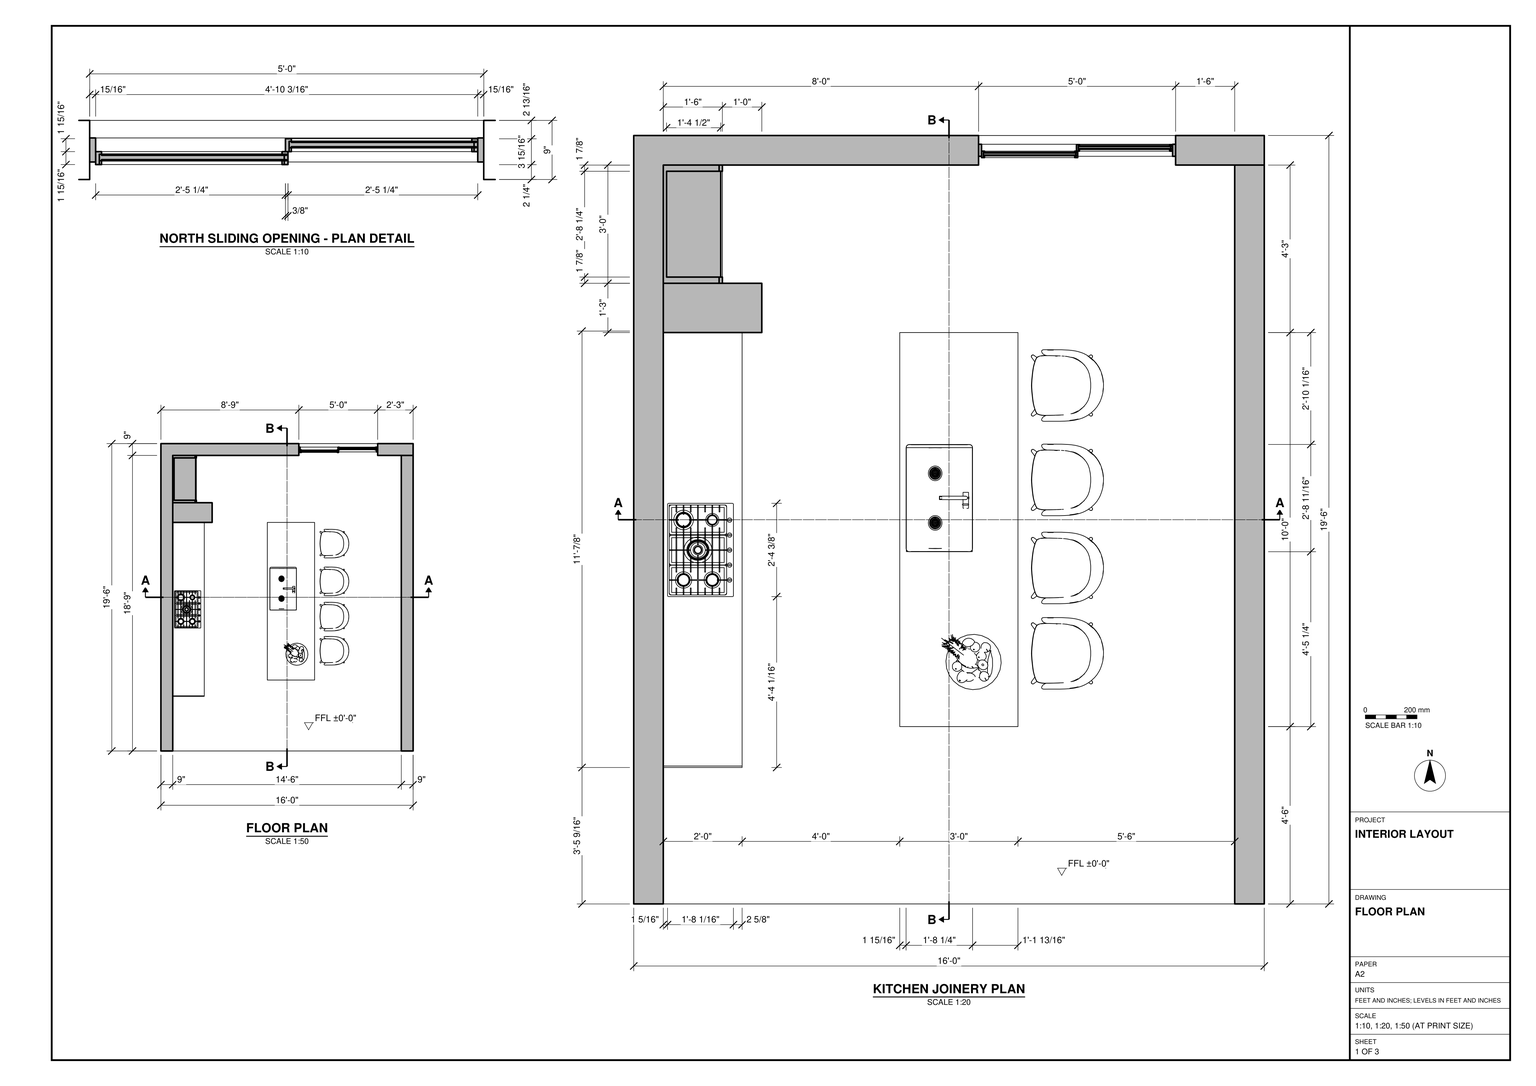
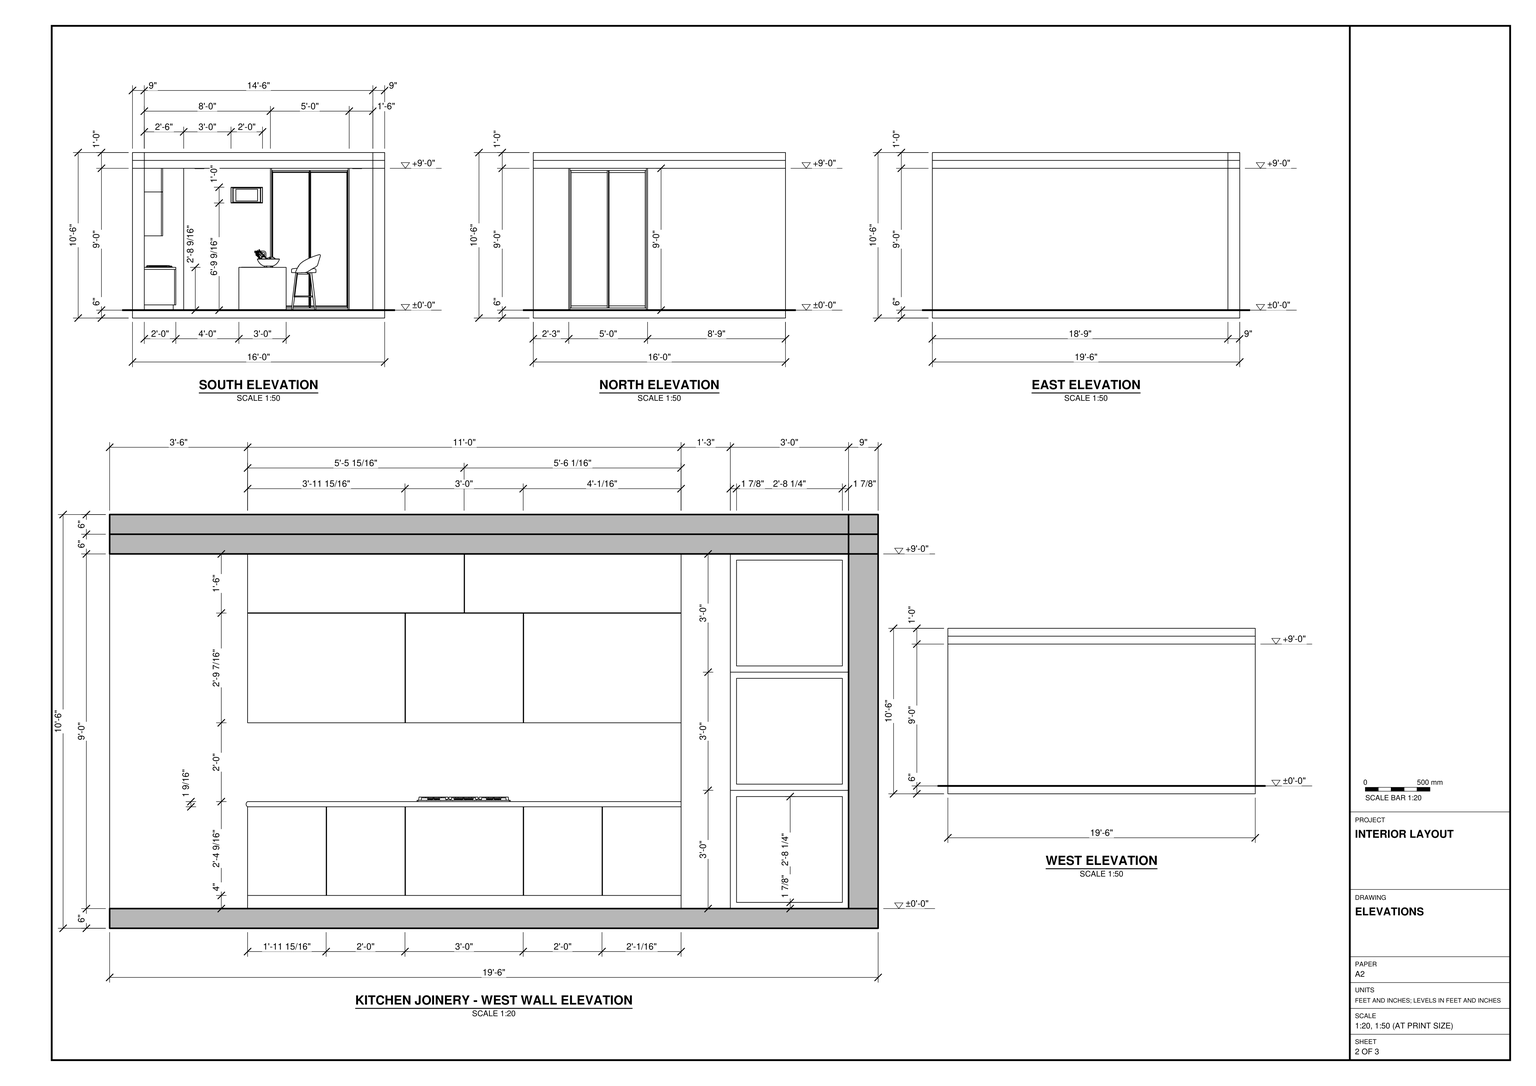
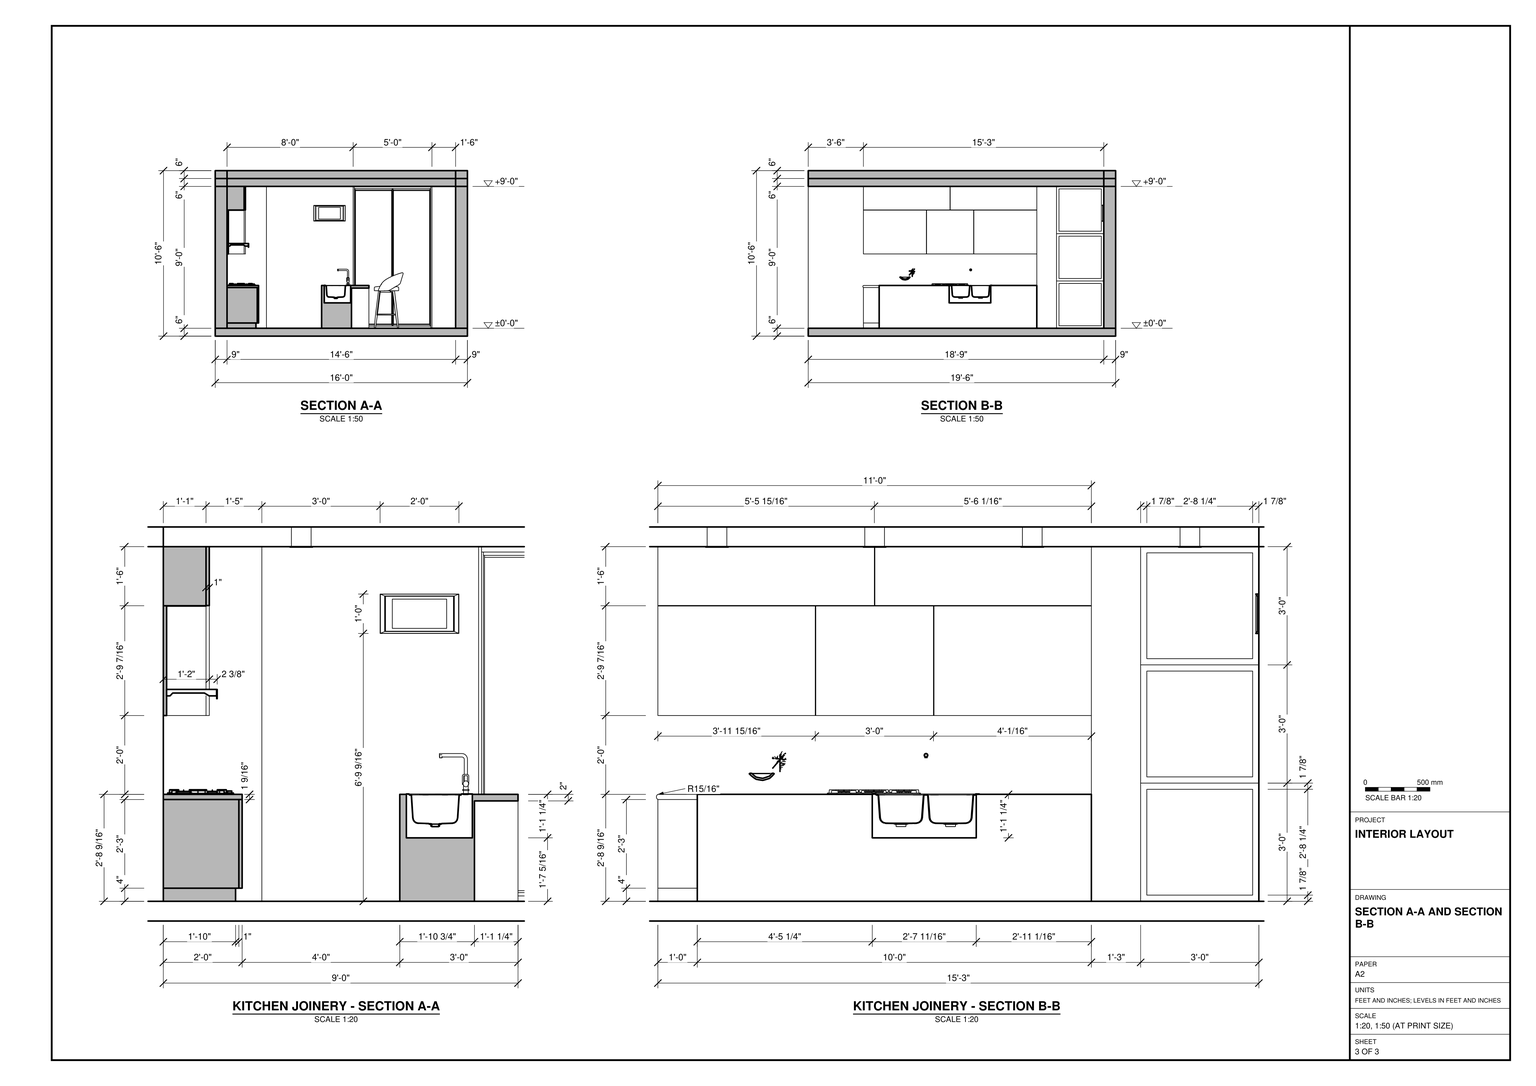
Use task_files/diagram_01.pdf to model the kitchen in SketchUp. Work in feet and inches. Set the finished floor at ±0'-0". The shell measures 16'-0" east to west by 19'-6" north to south and is 10'-6" high overall. Model the floor slab, the 9" walls on the west, north and east sides, and the flat ceiling and roof assembly shown in section. Leave the south side open. Use the enlarged plan detail for the two sliding panels in the north wall.

Build the west counter run with its recessed toe kick, divided cabinet fronts, cooktop and wall cabinets. Follow the west wall elevation for the two rows of upper cabinet fronts and the separate full-height storage at the north end. Set the island parallel to the counter, leaving a 4'-0" working aisle. Use the sections to position the double-bowl sink and tap and to form the overhang for the four stools on the east side. Place the fruit bowl near the south end of the island.

Keep the shell elements and each furniture or joinery piece in separate groups or components, and use components for repeated parts. Decor and loose items, including appliances, may be any suitable library components. Save one SketchUp model as output_files/kitchen_with_wall_cabinets_and_a_sink_island.skp.

# SketchUp Ruby script. Lengths in inches.
U = 1.inch
M = Sketchup.active_model
def pt(a) = Geom::Point3d.new(a.map { |v| v * U })
def face(e, loops, mat)
  f = e.add_face(loops[0].map { |a| pt(a) })
  loops[1..].each { |l| e.add_face(l.map { |a| pt(a) }).erase! }
  f.material = f.back_material = mat if mat
  f
end
# faces: each face lists its corners as indices into pts; further lists are holes
def faces(e, pts, list, mat = nil) = list.each { |f| face(e, (f[0].is_a?(Array) ? f : [f]).map { |l| l.map { |i| pts[i] } }, mat) }
# xy, xz, yz: faces in a plane at the given z, y or x. An outline is a flat list of corners, or four numbers for a rectangle; further outlines are holes
def ring(l) = l.size == 4 ? [[l[0], l[1]], [l[2], l[1]], [l[2], l[3]], [l[0], l[3]]] : l.each_slice(2).to_a
def flat(e, list, mat, &to3) = list.each { |f| face(e, (f[0].is_a?(Array) ? f : [f]).map { |l| ring(l).map { |u, v| to3.(u, v) } }, mat) }
def xy(e, z, list, mat = nil) = flat(e, list, mat) { |x, y| [x, y, z] }
def xz(e, y, list, mat = nil) = flat(e, list, mat) { |x, z| [x, y, z] }
def yz(e, x, list, mat = nil) = flat(e, list, mat) { |y, z| [x, y, z] }
def lines(e, pts, list) = list.each { |a, b| e.add_line(pt(pts[a]), pt(pts[b])) }
# prism: a flat outline (further loops are holes) pulled along v
def prism(e, loops, v, mat = nil)
  f = face(e, loops, mat); d = Geom::Vector3d.new(v.map { |x| x * U })
  f.pushpull(f.normal.samedirection?(d) ? d.length : -d.length)
end
def box(e, o, s, mat = nil) = prism(e, [[o, [o[0] + s[0], o[1], o[2]], [o[0] + s[0], o[1] + s[1], o[2]], [o[0], o[1] + s[1], o[2]]]], [0, 0, s[2]], mat)
def at(x, y, z, deg = 0) = Geom::Transformation.translation(pt([x, y, z])) * Geom::Transformation.rotation(ORIGIN, Z_AXIS, deg.degrees)
def axes(o, x, y, z) = Geom::Transformation.new([*x, 0, *y, 0, *z, 0, *pt(o).to_a, 1])
def part(name) = M.definitions.add(name)
# library, detail: a bought-in or finely detailed component or shape, given as its bounding box
def library(name, o, s) = part(name).tap { |d| box(d.entities, o, s) }
def detail(e, o, s) = box(e.add_group.entities, o, s)
def put(e, d, t, mat = nil) = e.add_instance(d, t).tap { |i| i.material = mat if mat }
def group(e, t, mat = nil) = e.add_group.tap { |g| g.transformation = t; g.material = mat if mat }.entities
root = M.entities
M.materials.add("Calacatta Marble (Y7X0XK)").color = [232, 232, 228]
M.materials.add("Charred Timber (ZWV9ZF)").color = [34, 34, 33]
M.materials.add("Resene FilmPro White -").color = [250, 246, 236]
M.materials.add("[0128_White]").color = [255, 255, 255]
M.materials.add("[0135_DarkGray]").color = [81, 81, 81]
M.materials.add("[Translucent Glass Gray]").color = [128, 128, 128]
M.materials["[Translucent Glass Gray]"].alpha = 0.5
M.materials.add("[Translucent Glass Gray]1").color = [128, 128, 128]
M.materials["[Translucent Glass Gray]1"].alpha = 0.15
c1 = library("Chimney",[0,-0.01,0],[29.73,15.52,29.75])
c2 = library("Piano cottura 702",[-24.9,5.55,2.1875],[20.06,28.4,1.39])
c3 = library("MIRELLA BAR HARD 7 colors",[-10.9,-9.34,0],[21.81,22.01,42.29])
c4 = library("Template",[-17.21,0.04,0.05],[27.44,26.51,14.69])
c5 = part("OA3")
g1 = group(c5.entities,at(77.64,-15.68,17.68))
prism(g1,[[[0.35,42.52,3.15],[0.35,42.52,51.84],[0.35,3.15,51.84],[0.35,3.15,3.15]],[[0.35,38.58,7.09],[0.35,7.09,7.09],[0.35,7.09,47.91],[0.35,38.58,47.91]]],[-0.35,0,0],"[0128_White]")
g2 = group(g1,at(1.57,0,0,90))
xy(g2,0,[[0,0,26.23,1.57],[26.23,0,45.67,1.57]],"Resene FilmPro White -")
xy(g2,0.2,[[0.2,0,45.47,0.12]],"Resene FilmPro White -")
xy(g2,2.64,[[2.64,0.71,43.03,0.83]],"Resene FilmPro White -")
xy(g2,2.76,[[2.76,0.83,42.91,0.94]],"Resene FilmPro White -")
xy(g2,3.03,[[3.03,0.94,42.64,1.0625]],"Resene FilmPro White -")
xy(g2,3.15,[[3.15,1.0625,42.52,1.57]],"Resene FilmPro White -")
xy(g2,51.84,[[3.15,1.0625,42.52,1.57]],"Resene FilmPro White -")
xy(g2,51.96,[[3.03,0.94,42.64,1.0625]],"Resene FilmPro White -")
xy(g2,52.24,[[2.76,0.83,42.91,0.94]],"Resene FilmPro White -")
xy(g2,52.35,[[2.64,0.71,43.03,0.83]],"Resene FilmPro White -")
xy(g2,54.8,[[0.2,0,45.47,0.12]],"Resene FilmPro White -")
xy(g2,54.99,[[0,0,45.67,1.57]],"Resene FilmPro White -")
xz(g2,0,[[[0,0,45.67,54.99],[0.2,0.2,45.47,54.8]]],"Resene FilmPro White -")
xz(g2,0.83,[[[2.64,2.64,43.03,52.35],[2.76,2.76,42.91,52.24]]],"Resene FilmPro White -")
xz(g2,0.94,[[[2.76,2.76,42.91,52.24],[3.03,3.03,42.64,51.96]]],"Resene FilmPro White -")
xz(g2,1.0625,[[[3.03,3.03,42.64,51.96],[3.15,3.15,42.52,51.84]]],"Resene FilmPro White -")
xz(g2,1.57,[[[0,0,45.67,54.99],[3.15,3.15,42.52,51.84]]],"Resene FilmPro White -")
yz(g2,0,[[0,0,1.57,54.99]],"Resene FilmPro White -")
yz(g2,0.2,[[0,0.2,0.12,54.8]],"Resene FilmPro White -")
yz(g2,2.64,[[0.71,2.64,0.83,52.35]],"Resene FilmPro White -")
yz(g2,2.76,[[0.83,2.76,0.94,52.24]],"Resene FilmPro White -")
yz(g2,3.03,[[0.94,3.03,1.0625,51.96]],"Resene FilmPro White -")
yz(g2,3.15,[[1.0625,3.15,1.57,51.84]],"Resene FilmPro White -")
yz(g2,42.52,[[1.0625,3.15,1.57,51.84]],"Resene FilmPro White -")
yz(g2,42.64,[[0.94,3.03,1.0625,51.96]],"Resene FilmPro White -")
yz(g2,42.91,[[0.83,2.76,0.94,52.24]],"Resene FilmPro White -")
yz(g2,43.03,[[0.71,2.64,0.83,52.35]],"Resene FilmPro White -")
yz(g2,45.47,[[0,0.2,0.12,54.8]],"Resene FilmPro White -")
yz(g2,45.67,[[0,0,1.57,54.99]],"Resene FilmPro White -")
p = [[2.64,0.71,52.35],[0.2,0.12,54.8],[0.2,0.12,0.2],[2.64,0.71,2.64],[45.47,0.12,0.2],[43.03,0.71,2.64],
  [45.47,0.12,54.8],[43.03,0.71,52.35]]
faces(g2,p,[[0,1,2,3],[3,2,4,5],[5,4,6,7],[7,6,1,0]],"Resene FilmPro White -")
c6 = library("sink",[0,0,0],[20.24,32.66,22.26])
c7 = part("PENTEK_RP Fineline 50S_Sliding_DoorCase_E1")
box(c7.entities,[0,0,0],[1.51,3.66,99.27],"[0135_DarkGray]")
c8 = part("PENTEK_RP Fineline 50S_SlidingDooe_Case_E2")
box(c8.entities,[0,0,0],[96.25,3.66,1.51],"[0135_DarkGray]")
c9 = part("pentek_RP Fineline 50S_SlidingDoor_Case")
put(c9.entities,c7,at(97.76,0,0))
put(c9.entities,c8,at(1.51,0,0))
put(c9.entities,c7,at(0,0,0))
put(c9.entities,c8,at(1.51,0,97.76))
c10 = part("PENTEK_RP Fineline 50S_SlidingDoor_GlazingBead_2")
box(c10.entities,[0,0,0],[0.56,0.59,94.39],"[0135_DarkGray]")
c11 = part("PENTEK_RP Fineline 50S_SlidingDoor_Glass")
box(c11.entities,[0,0,0],[46.58,0.16,94.39],"[Translucent Glass Gray]1")
c12 = part("PENTEK_RP Fineline 50S_SlidingDoor_GlazingBead")
box(c12.entities,[0,0,0],[45.47,0.59,0.56],"[0135_DarkGray]")
c13 = part("PENTEK_RP Fineline 50S_SlidingDoor_Leaf_E1")
xy(c13.entities,0,[[0,0,0.93,1.97],[0.93,1.57,1.49,1.97]],"[0135_DarkGray]")
xy(c13.entities,96.25,[[0,0,0.93,0,0.93,1.57,1.49,1.57,1.49,1.97,0,1.97]],"[0135_DarkGray]")
xz(c13.entities,0,[[0,0,0.93,96.25]],"[0135_DarkGray]")
xz(c13.entities,1.57,[[0.93,0,1.49,95.32],[0.93,95.32,1.49,96.25]],"[0135_DarkGray]")
xz(c13.entities,1.97,[[0,0,1.49,96.25]],"[0135_DarkGray]")
yz(c13.entities,0,[[0,0,1.97,96.25]],"[0135_DarkGray]")
yz(c13.entities,0.93,[[0,0,1.57,0.93],[0,0.93,1.57,95.32],[0,95.32,1.57,96.25]],"[0135_DarkGray]")
yz(c13.entities,1.49,[[1.57,0,1.97,95.32],[1.57,95.32,1.97,96.25]],"[0135_DarkGray]")
c14 = part("PENTEK_RP Fineline 50S_SlidingDoor_Leaf_E2")
xy(c14.entities,0,[[0,0,0,1.57,0.56,1.57,0.56,1.97,46.02,1.97,46.02,1.57,46.58,1.57,46.58,0]],"[0135_DarkGray]")
xy(c14.entities,0.93,[[0,0,46.58,1.57]],"[0135_DarkGray]")
xy(c14.entities,1.49,[[0.56,1.57,46.02,1.97]],"[0135_DarkGray]")
xz(c14.entities,0,[[0,0,46.58,0.93]],"[0135_DarkGray]")
xz(c14.entities,1.57,[[0,0,0.56,0.93],[46.02,0,46.58,0.93],[0.56,0.93,46.02,1.49]],"[0135_DarkGray]")
xz(c14.entities,1.97,[[0.56,0,46.02,1.49]],"[0135_DarkGray]")
yz(c14.entities,0,[[0,0,1.57,0.93]],"[0135_DarkGray]")
yz(c14.entities,0.56,[[1.57,0,1.97,0.93],[1.57,0.93,1.97,1.49]],"[0135_DarkGray]")
yz(c14.entities,46.02,[[1.57,0,1.97,0.93],[1.57,0.93,1.97,1.49]],"[0135_DarkGray]")
yz(c14.entities,46.58,[[0,0,1.57,0.93]],"[0135_DarkGray]")
c15 = part("PENTEK_RP Fineline S_SlidingDoor_Leaf1")
put(c15.entities,c10,at(0.93,0,0.93))
put(c15.entities,c10,at(46.96,0,0.93))
put(c15.entities,c11,at(1.49,1.42,0.93))
put(c15.entities,c12,at(1.49,0,0.93))
put(c15.entities,c11,at(1.49,0.59,0.93))
put(c15.entities,c13,at(0,0,0))
put(c15.entities,c13,axes([48.44,0,0],[-1,0,0],[0,1,0],[0,0,1]))
put(c15.entities,c14,axes([0.93,0,96.25],[1,0,0],[0,1,0],[0,0,-1]))
put(c15.entities,c14,at(0.93,0,0))
put(c15.entities,c12,at(1.49,0,94.77))
c16 = part("PENTEK_RP Fineline 50S_SlidingDoor_Leaf2")
put(c16.entities,c11,at(1.49,1.42,0.93))
put(c16.entities,c12,at(1.49,0,94.77))
put(c16.entities,c10,at(46.96,0,0.93))
put(c16.entities,c11,at(1.49,0.59,0.93))
put(c16.entities,c10,at(0.93,0,0.93))
put(c16.entities,c13,at(0,0,0))
put(c16.entities,c13,axes([48.44,0,0],[-1,0,0],[0,1,0],[0,0,1]))
put(c16.entities,c12,at(1.49,0,0.93))
put(c16.entities,c14,axes([0.93,0,96.25],[1,0,0],[0,1,0],[0,0,-1]))
put(c16.entities,c14,at(0.93,0,0))
c17 = part("PENTEK_RP+Fineline+50S_Sliding_Door+(1)")
put(c17.entities,c9,at(0,-1.88,-0.09))
put(c17.entities,c15,at(1.51,-2.27,1.42))
put(c17.entities,c16,at(49.32,-0.3,1.42))
c18 = part("Side plate")
xy(c18.entities,-0.25,[[[2.99,-0.5,2.09,-0.38,1.24,-0.03,0.52,0.53,-0.03,1.26,-0.38,2.1,-0.5,3.01,-0.38,3.91,-0.03,4.76,0.53,5.48,1.26,6.03,2.1,6.38,3.01,6.5,3.91,6.38,4.76,6.03,5.48,5.47,6.03,4.74,6.38,3.9,6.5,2.99,6.38,2.09,6.03,1.24,5.47,0.52,4.74,-0.03,3.9,-0.38],[2.99,0,3.77,0.1,4.49,0.4,5.12,0.875,5.6,1.49,5.9,2.22,6,2.99,5.9,3.77,5.6,4.49,5.125,5.12,4.51,5.6,3.78,5.9,3.01,6,2.23,5.9,1.51,5.6,0.88,5.125,0.4,4.51,0.1,3.78,0,3.01,0.1,2.23,0.4,1.51,0.875,0.88,1.49,0.4,2.22,0.1]]])
xy(c18.entities,0,[[[2.99,-0.5,3.9,-0.38,4.74,-0.03,5.47,0.52,6.03,1.24,6.38,2.09,6.5,2.99,6.38,3.9,6.03,4.74,5.48,5.47,4.76,6.03,3.91,6.38,3.01,6.5,2.1,6.38,1.26,6.03,0.53,5.48,-0.03,4.76,-0.38,3.91,-0.5,3.01,-0.38,2.1,-0.03,1.26,0.52,0.53,1.24,-0.03,2.09,-0.38],[2.99,0,2.22,0.1,1.49,0.4,0.875,0.88,0.4,1.51,0.1,2.23,0,3.01,0.1,3.78,0.4,4.51,0.88,5.125,1.51,5.6,2.23,5.9,3.01,6,3.78,5.9,4.51,5.6,5.125,5.12,5.6,4.49,5.9,3.77,6,2.99,5.9,2.22,5.6,1.49,5.12,0.875,4.49,0.4,3.77,0.1]],[2.99,0,3.77,0.1,4.49,0.4,5.12,0.875,5.6,1.49,5.9,2.22,6,2.99,5.9,3.77,5.6,4.49,5.125,5.12,4.51,5.6,3.78,5.9,3.01,6,2.23,5.9,1.51,5.6,0.88,5.125,0.4,4.51,0.1,3.78,0,3.01,0.1,2.23,0.4,1.51,0.875,0.88,1.49,0.4,2.22,0.1]])
p = [[2.99,-0.5,0],[2.09,-0.38,0],[2.09,-0.38,-0.25],[2.99,-0.5,-0.25],[3.9,-0.38,0],[3.9,-0.38,-0.25],
  [1.24,-0.03,0],[1.24,-0.03,-0.25],[4.74,-0.03,0],[4.74,-0.03,-0.25],[0.52,0.53,0],[0.52,0.53,-0.25],
  [2.22,0.1,0],[2.99,0,0],[2.99,0,-0.25],[2.22,0.1,-0.25],[3.77,0.1,0],[3.77,0.1,-0.25],
  [5.47,0.52,0],[5.47,0.52,-0.25],[1.49,0.4,0],[1.49,0.4,-0.25],[4.49,0.4,0],[4.49,0.4,-0.25],
  [0.875,0.88,0],[0.875,0.88,-0.25],[5.12,0.875,0],[5.12,0.875,-0.25],[-0.03,1.26,0],[-0.03,1.26,-0.25],
  [6.03,1.24,0],[6.03,1.24,-0.25],[0.4,1.51,0],[0.4,1.51,-0.25],[5.6,1.49,0],[5.6,1.49,-0.25],
  [6.38,2.09,0],[6.38,2.09,-0.25],[-0.38,2.1,0],[-0.38,2.1,-0.25],[0.1,2.23,0],[0.1,2.23,-0.25],
  [5.9,2.22,0],[5.9,2.22,-0.25],[-0.5,3.01,0],[-0.5,3.01,-0.25],[6.5,2.99,0],[6.5,2.99,-0.25],
  [0,3.01,0],[0,3.01,-0.25],[6,2.99,0],[6,2.99,-0.25],[-0.38,3.91,0],[-0.38,3.91,-0.25],
  [0.1,3.78,0],[0.1,3.78,-0.25],[5.9,3.77,0],[5.9,3.77,-0.25],[6.38,3.9,0],[6.38,3.9,-0.25],
  [0.4,4.51,0],[0.4,4.51,-0.25],[5.6,4.49,0],[5.6,4.49,-0.25],[-0.03,4.76,0],[-0.03,4.76,-0.25],
  [6.03,4.74,0],[6.03,4.74,-0.25],[0.88,5.125,0],[0.88,5.125,-0.25],[5.125,5.12,0],[5.125,5.12,-0.25],
  [5.48,5.47,0],[5.48,5.47,-0.25],[0.53,5.48,0],[0.53,5.48,-0.25],[1.51,5.6,0],[1.51,5.6,-0.25],
  [4.51,5.6,0],[4.51,5.6,-0.25],[1.26,6.03,0],[1.26,6.03,-0.25],[4.76,6.03,0],[4.76,6.03,-0.25],
  [2.23,5.9,0],[2.23,5.9,-0.25],[3.78,5.9,0],[3.78,5.9,-0.25],[3.01,6,0],[3.01,6,-0.25],
  [2.1,6.38,0],[2.1,6.38,-0.25],[3.91,6.38,0],[3.91,6.38,-0.25],[3.01,6.5,0],[3.01,6.5,-0.25]]
faces(c18.entities,p,[[0,1,2,3],[4,0,3,5],[1,6,7,2],[8,4,5,9],[6,10,11,7],[12,13,14,15],[13,16,17,14],[18,8,9,19],
  [20,12,15,21],[16,22,23,17],[24,20,21,25],[22,26,27,23],[10,28,29,11],[30,18,19,31],[32,24,25,33],[26,34,35,27],
  [36,30,31,37],[28,38,39,29],[40,32,33,41],[34,42,43,35],[38,44,45,39],[46,36,37,47],[48,40,41,49],[42,50,51,43],
  [44,52,53,45],[54,48,49,55],[50,56,57,51],[58,46,47,59],[60,54,55,61],[56,62,63,57],[52,64,65,53],[66,58,59,67],
  [68,60,61,69],[62,70,71,63],[72,66,67,73],[64,74,75,65],[76,68,69,77],[70,78,79,71],[74,80,81,75],[82,72,73,83],
  [84,76,77,85],[78,86,87,79],[88,84,85,89],[86,88,89,87],[80,90,91,81],[92,82,83,93],[90,94,95,91],[94,92,93,95]])
c19 = part("Group\#20")
box(c19.entities,[0,-42,0],[192,234,6])
c20 = part("Group\#17")
yz(c20.entities,0,[[0,0,32.23,32.23]])
p = [[105,225,114],[105,225,6],[165,225,6],[165,225,114]]
lines(root,p,[[0,1],[1,2],[2,3],[3,0]])
put(root,c1,at(25.46,93.36,66.17,90))
put(root,c2,at(5.45,127.54,36.39,-180))
put(root,c3,at(130.38,76.31,6,-90))
put(root,c3,at(130.38,102.31,6,-90))
put(root,c3,at(130.38,129.12,6,-90))
put(root,c3,at(130.38,157.87,6,-90))
put(root,c4,at(104.99,61.89,38.57))
put(root,c5,axes([83.24,270.81,83.71],[0,-0.59,0],[0.52552,0,0],[0,0,0.21821]))
put(root,c6,at(103.17,139.91,28.74,-180))
put(root,c17,axes([105,229.55,6.1],[0.6044,0,0],[0,1,0],[0,0,1.08792]))
put(root,c18,at(168,9,114))
put(root,c18,at(168,57,114))
put(root,c18,at(168,105,114))
put(root,c18,at(168,153,114))
put(root,c18,at(168,201,114))
put(root,c18,at(48,201,114))
put(root,c18,at(48,153,114))
put(root,c18,at(48,105,114))
put(root,c18,at(48,57,114))
put(root,c18,at(48,9,114))
put(root,c19,at(0,42,0))
g3 = group(root,at(0,42,6),"Calacatta Marble (Y7X0XK)")
xy(g3,0,[[0,-42,0,192,105,192,105,183,9,183,9,-42],[165,183,192,192]])
xy(g3,108,[[105,183,165,192]])
xy(g3,120,[[0,-42,9,-42,9,183,192,183,192,192,0,192]])
xz(g3,-42,[[0,0,9,120]])
xz(g3,183,[[9,0,105,0,105,108,165,108,165,0,192,0,192,120,9,120]])
xz(g3,192,[[0,0,0,120,192,120,192,0,165,0,165,108,105,108,105,0]])
yz(g3,0,[[-42,0,192,120]])
yz(g3,9,[[-42,0,183,120]])
yz(g3,105,[[183,0,192,108]])
yz(g3,165,[[183,0,192,108]])
yz(g3,192,[[183,0,192,120]])
g4 = group(root,at(183,42,6))
box(g4,[0,-42,0],[9,225,120])
g5 = group(root,at(9,42,6),"Calacatta Marble (Y7X0XK)")
box(g5,[0,0,0],[22,132,4])
g6 = group(root,at(9,42,10))
box(g6,[0,0,0],[23,132,27])
g7 = group(root,at(9,42,37),"Calacatta Marble (Y7X0XK)")
xy(g7,0,[[0,0,24,132]])
xy(g7,1.57,[[0,0,24,132]])
yz(g7,0,[[0,0,-0.13,0.09,-0.24,0.2,-0.33,0.33,-0.4,0.48,-0.4375,0.63,-0.45,0.79,-0.4375,0.95,-0.4,1.1,-0.33,1.24,-0.24,1.37,-0.13,1.48,0,1.57],[0,0,132,1.57],[132,0,132,1.57,132.125,1.48,132.23,1.37,132.32,1.24,132.39,1.09,132.42,0.94,132.4375,0.79,132.42,0.63,132.39,0.48,132.32,0.34,132.23,0.21,132.125,0.09]])
yz(g7,24,[[0,0,132,0,132.125,0.09,132.23,0.21,132.32,0.34,132.39,0.48,132.42,0.63,132.4375,0.79,132.42,0.94,132.39,1.09,132.32,1.24,132.23,1.37,132.125,1.48,132,1.57,0,1.57,-0.13,1.48,-0.24,1.37,-0.33,1.24,-0.4,1.1,-0.4375,0.95,-0.45,0.79,-0.4375,0.63,-0.4,0.48,-0.33,0.33,-0.24,0.2,-0.13,0.09]])
p = [[24,0,0],[24,-0.13,0.09],[0,-0.13,0.09],[0,0,0],[24,132.125,0.09],[24,132,0],
  [0,132,0],[0,132.125,0.09],[24,-0.24,0.2],[0,-0.24,0.2],[24,132.23,0.21],[0,132.23,0.21],
  [24,-0.33,0.33],[0,-0.33,0.33],[24,132.32,0.34],[0,132.32,0.34],[24,-0.4,0.48],[0,-0.4,0.48],
  [24,132.39,0.48],[0,132.39,0.48],[24,-0.4375,0.63],[0,-0.4375,0.63],[24,132.42,0.63],[0,132.42,0.63],
  [24,-0.45,0.79],[0,-0.45,0.79],[24,132.4375,0.79],[0,132.4375,0.79],[24,-0.4375,0.95],[0,-0.4375,0.95],
  [24,132.42,0.94],[0,132.42,0.94],[24,-0.4,1.1],[0,-0.4,1.1],[24,132.39,1.09],[0,132.39,1.09],
  [24,-0.33,1.24],[0,-0.33,1.24],[24,132.32,1.24],[0,132.32,1.24],[24,-0.24,1.37],[0,-0.24,1.37],
  [24,132.23,1.37],[0,132.23,1.37],[24,-0.13,1.48],[0,-0.13,1.48],[24,132.125,1.48],[0,132.125,1.48],
  [24,0,1.57],[0,0,1.57],[24,132,1.57],[0,132,1.57]]
faces(g7,p,[[0,1,2,3],[4,5,6,7],[1,8,9,2],[10,4,7,11],[8,12,13,9],[14,10,11,15],[12,16,17,13],[18,14,15,19],
  [16,20,21,17],[22,18,19,23],[20,24,25,21],[26,22,23,27],[24,28,29,25],[30,26,27,31],[28,32,33,29],[34,30,31,35],
  [32,36,37,33],[38,34,35,39],[36,40,41,37],[42,38,39,43],[40,44,45,41],[46,42,43,47],[44,48,49,45],[50,46,47,51]])
g8 = group(root,at(32,42,10))
xy(g8,0,[[0,0,1,23.92],[0,24.08,1,47.92],[0,48.08,1,83.92],[0,84.08,1,107.92],[0,108.08,1,132]])
xy(g8,27,[[0,0,1,23.92],[0,24.08,1,47.92],[0,48.08,1,83.92],[0,84.08,1,107.92],[0,108.08,1,132]])
xz(g8,0,[[0,0,1,27]])
xz(g8,23.92,[[0,0,1,27]])
xz(g8,24.08,[[0,0,1,27]])
xz(g8,47.92,[[0,0,1,27]])
xz(g8,48.08,[[0,0,1,27]])
xz(g8,83.92,[[0,0,1,27]])
xz(g8,84.08,[[0,0,1,27]])
xz(g8,107.92,[[0,0,1,27]])
xz(g8,108.08,[[0,0,1,27]])
xz(g8,132,[[0,0,1,27]])
yz(g8,0,[[0,0,23.92,27],[23.92,0,24.08,27],[24.08,0,47.92,27],[47.92,0,48.08,27],[48.08,0,83.92,27],
  [83.92,0,84.08,27],[84.08,0,107.92,27],[107.92,0,108.08,27],[108.08,0,132,27]])
yz(g8,1,[[0,0,23.92,27],[24.08,0,47.92,27],[48.08,0,83.92,27],[84.08,0,107.92,27],[108.08,0,132,27]])
g9 = group(root,at(9,42,96),"Charred Timber (ZWV9ZF)")
box(g9,[0,0,0],[13,132,18])
g10 = group(root,at(22,42,96),"Charred Timber (ZWV9ZF)")
xy(g10,0.08,[[0,0,1,65.92],[0,66.08,1,132]])
xy(g10,18,[[0,0,1,65.92],[0,66.08,1,132]])
xz(g10,0,[[0,0.08,1,18]])
xz(g10,65.92,[[0,0.08,1,18]])
xz(g10,66.08,[[0,0.08,1,18]])
xz(g10,132,[[0,0.08,1,18]])
yz(g10,0,[[65.92,0,66.08,18],[0,0.08,65.92,18],[66.08,0.08,132,18]])
yz(g10,1,[[0,0.08,65.92,18],[66.08,0.08,132,18]])
g11 = group(root,at(9,42,62.57),"Charred Timber (ZWV9ZF)")
xy(g11,0,[[0,0,0,132,13,132,13,83.92,1,83.92,1,48.08,13,48.08,13,0]])
xy(g11,33.35,[[1,48.08,13,83.92]])
xy(g11,33.43,[[0,0,13,132]])
xz(g11,0,[[0,0,13,33.43]])
xz(g11,48.08,[[1,0,13,33.35]])
xz(g11,83.92,[[1,0,13,33.35]])
xz(g11,132,[[0,0,13,33.43]])
yz(g11,0,[[0,0,132,33.43]])
yz(g11,1,[[48.08,0,83.92,33.35]])
yz(g11,13,[[0,0,48.08,0,48.08,33.35,83.92,33.35,83.92,0,132,0,132,33.43,0,33.43]])
g12 = group(root,at(22,42,62.57),"Charred Timber (ZWV9ZF)")
xy(g12,0,[[0,0,1,47.92],[0,84.08,1,132]])
xy(g12,33.35,[[0,0,1,47.92],[0,84.08,1,132]])
xz(g12,0,[[0,0,1,33.35]])
xz(g12,47.92,[[0,0,1,33.35]])
xz(g12,84.08,[[0,0,1,33.35]])
xz(g12,132,[[0,0,1,33.35]])
yz(g12,0,[[0,0,47.92,33.35],[47.92,0,48.08,33.35],[83.92,0,84.08,33.35],[84.08,0,132,33.35]])
yz(g12,1,[[0,0,47.92,33.35],[84.08,0,132,33.35]])
p = [[1,65.92,33.5],[1,65.92,33.35],[1,66.08,33.5],[1,66.08,33.35]]
lines(g12,p,[[0,1],[2,3]])
g13 = group(root,at(9,174,6))
box(g13,[0,0,0],[30,15,108])
g14 = group(root,at(81,54,6),"Calacatta Marble (Y7X0XK)")
xy(g14,0,[[0,0,0,120,36,120,36,118,22.74,118,22.74,2,36,2,36,0]])
xy(g14,19.32,[[2.01,53.28,22.1,84.94]])
xy(g14,30.57,[[22.74,2,36,118]])
xy(g14,32.57,[[[0,0,36,120],[2.01,53.28,22.1,84.94]]])
xz(g14,0,[[0,0,36,32.57]])
xz(g14,2,[[22.74,0,36,30.57]])
xz(g14,53.28,[[2.01,19.32,22.1,32.57]])
xz(g14,84.94,[[2.01,19.32,22.1,32.57]])
xz(g14,118,[[22.74,0,36,30.57]])
xz(g14,120,[[0,0,36,32.57]])
yz(g14,0,[[0,0,120,32.57]])
yz(g14,2.01,[[53.28,19.32,84.94,32.57]])
yz(g14,22.1,[[53.28,19.32,84.94,32.57]])
yz(g14,22.74,[[2,0,118,30.57]])
yz(g14,36,[[0,0,2,0,2,30.57,118,30.57,118,0,120,0,120,32.57,0,32.57]])
g15 = group(root,at(9,189,6))
xy(g15,0,[[0,0,17,36]])
xy(g15,1.89,[[1,1.89,17,34.11]])
xy(g15,34.11,[[1,1.89,17,34.11]])
xy(g15,37.89,[[1,1.89,17,34.11]])
xy(g15,70.11,[[1,1.89,17,34.11]])
xy(g15,73.89,[[1,1.89,17,34.11]])
xy(g15,106.11,[[1,1.89,17,34.11]])
xy(g15,108,[[0,0,17,36]])
xz(g15,0,[[0,0,17,108]])
xz(g15,1.89,[[1,1.89,17,34.11],[1,37.89,17,70.11],[1,73.89,17,106.11]])
xz(g15,34.11,[[1,1.89,17,34.11],[1,37.89,17,70.11],[1,73.89,17,106.11]])
xz(g15,36,[[0,0,17,108]])
yz(g15,0,[[0,0,36,108]])
yz(g15,1,[[1.89,1.89,34.11,34.11],[1.89,37.89,34.11,70.11],[1.89,73.89,34.11,106.11]])
yz(g15,17,[[[0,0,36,108],[1.89,73.89,34.11,106.11],[1.89,37.89,34.11,70.11],[1.89,1.89,34.11,34.11]]])
g16 = group(root,at(26,189,6))
xy(g16,0,[[0,0,1,36]])
xy(g16,1.89,[[0,1.89,1,34.11]])
xy(g16,34.11,[[0,1.89,1,34.11]])
xy(g16,37.89,[[0,1.89,1,34.11]])
xy(g16,70.11,[[0,1.89,1,34.11]])
xy(g16,73.89,[[0,1.89,0.5,34.11],[0.5,1.89,1,34.11]])
xy(g16,106.11,[[0,1.89,0.5,34.11],[0.5,1.89,1,34.11]])
xy(g16,108,[[0,0,1,36]])
xz(g16,0,[[0,0,1,108]])
xz(g16,1.89,[[0,1.89,1,34.11],[0,37.89,1,70.11],[0,73.89,0.5,106.11],[0.5,73.89,1,106.11]])
xz(g16,34.11,[[0,1.89,1,34.11],[0,37.89,1,70.11],[0,73.89,0.5,106.11],[0.5,73.89,1,106.11]])
xz(g16,36,[[0,0,1,108]])
yz(g16,0,[[[0,0,36,108],[1.89,73.89,34.11,106.11],[1.89,37.89,34.11,70.11],[1.89,1.89,34.11,34.11]]])
yz(g16,1,[[[0,0,36,36],[1.89,1.89,34.11,34.11]],[[0,36,36,72],[1.89,37.89,34.11,70.11]],[[0,72,36,108],[1.89,73.89,34.11,106.11]]])
g17 = group(g16,at(0.5,1.89,73.89),"[Translucent Glass Gray]")
yz(g17,0,[[0,0,32.23,32.23]])
put(g16,c20,at(0.5,1.89,37.89),"[Translucent Glass Gray]")
put(g16,c20,at(0.5,1.89,1.89),"[Translucent Glass Gray]")
put(root,c19,at(0,42,120))
g18 = group(root,at(0,42,114))
prism(g18,[[[0,-42,0],[0,192,0],[192,192,0],[192,-42,0]],[[168,66.01,0],[168.1,65.23,0],[168.4,64.51,0],[168.875,63.88,0],[169.49,63.4,0],[170.22,63.1,0],[170.99,63,0],[171.77,63.1,0],[172.49,63.4,0],[173.12,63.875,0],[173.6,64.49,0],[173.9,65.22,0],[174,65.99,0],[173.9,66.77,0],[173.6,67.49,0],[173.125,68.12,0],[172.51,68.6,0],[171.78,68.9,0],[171.01,69,0],[170.23,68.9,0],[169.51,68.6,0],[168.88,68.125,0],[168.4,67.51,0],[168.1,66.78,0]],[[170.99,-33,0],[171.77,-32.9,0],[172.49,-32.6,0],[173.12,-32.125,0],[173.6,-31.51,0],[173.9,-30.78,0],[174,-30.01,0],[173.9,-29.23,0],[173.6,-28.51,0],[173.125,-27.88,0],[172.51,-27.4,0],[171.78,-27.1,0],[171.01,-27,0],[170.23,-27.1,0],[169.51,-27.4,0],[168.88,-27.875,0],[168.4,-28.49,0],[168.1,-29.22,0],[168,-29.99,0],[168.1,-30.77,0],[168.4,-31.49,0],[168.875,-32.12,0],[169.49,-32.6,0],[170.22,-32.9,0]],[[168,18.01,0],[168.1,17.23,0],[168.4,16.51,0],[168.875,15.88,0],[169.49,15.4,0],[170.22,15.1,0],[170.99,15,0],[171.77,15.1,0],[172.49,15.4,0],[173.12,15.875,0],[173.6,16.49,0],[173.9,17.22,0],[174,17.99,0],[173.9,18.77,0],[173.6,19.49,0],[173.125,20.12,0],[172.51,20.6,0],[171.78,20.9,0],[171.01,21,0],[170.23,20.9,0],[169.51,20.6,0],[168.88,20.125,0],[168.4,19.51,0],[168.1,18.78,0]],[[168,114.01,0],[168.1,113.23,0],[168.4,112.51,0],[168.875,111.88,0],[169.49,111.4,0],[170.22,111.1,0],[170.99,111,0],[171.77,111.1,0],[172.49,111.4,0],[173.12,111.875,0],[173.6,112.49,0],[173.9,113.22,0],[174,113.99,0],[173.9,114.77,0],[173.6,115.49,0],[173.125,116.12,0],[172.51,116.6,0],[171.78,116.9,0],[171.01,117,0],[170.23,116.9,0],[169.51,116.6,0],[168.88,116.125,0],[168.4,115.51,0],[168.1,114.78,0]],[[168,162.01,0],[168.1,161.23,0],[168.4,160.51,0],[168.875,159.88,0],[169.49,159.4,0],[170.22,159.1,0],[170.99,159,0],[171.77,159.1,0],[172.49,159.4,0],[173.12,159.875,0],[173.6,160.49,0],[173.9,161.22,0],[174,161.99,0],[173.9,162.77,0],[173.6,163.49,0],[173.125,164.12,0],[172.51,164.6,0],[171.78,164.9,0],[171.01,165,0],[170.23,164.9,0],[169.51,164.6,0],[168.88,164.125,0],[168.4,163.51,0],[168.1,162.78,0]],[[48,162.01,0],[48.1,161.23,0],[48.4,160.51,0],[48.875,159.88,0],[49.49,159.4,0],[50.22,159.1,0],[50.99,159,0],[51.77,159.1,0],[52.49,159.4,0],[53.12,159.875,0],[53.6,160.49,0],[53.9,161.22,0],[54,161.99,0],[53.9,162.77,0],[53.6,163.49,0],[53.125,164.12,0],[52.51,164.6,0],[51.78,164.9,0],[51.01,165,0],[50.23,164.9,0],[49.51,164.6,0],[48.88,164.125,0],[48.4,163.51,0],[48.1,162.78,0]],[[48,114.01,0],[48.1,113.23,0],[48.4,112.51,0],[48.875,111.88,0],[49.49,111.4,0],[50.22,111.1,0],[50.99,111,0],[51.77,111.1,0],[52.49,111.4,0],[53.12,111.875,0],[53.6,112.49,0],[53.9,113.22,0],[54,113.99,0],[53.9,114.77,0],[53.6,115.49,0],[53.125,116.12,0],[52.51,116.6,0],[51.78,116.9,0],[51.01,117,0],[50.23,116.9,0],[49.51,116.6,0],[48.88,116.125,0],[48.4,115.51,0],[48.1,114.78,0]],[[48,66.01,0],[48.1,65.23,0],[48.4,64.51,0],[48.875,63.88,0],[49.49,63.4,0],[50.22,63.1,0],[50.99,63,0],[51.77,63.1,0],[52.49,63.4,0],[53.12,63.875,0],[53.6,64.49,0],[53.9,65.22,0],[54,65.99,0],[53.9,66.77,0],[53.6,67.49,0],[53.125,68.12,0],[52.51,68.6,0],[51.78,68.9,0],[51.01,69,0],[50.23,68.9,0],[49.51,68.6,0],[48.88,68.125,0],[48.4,67.51,0],[48.1,66.78,0]],[[48,18.01,0],[48.1,17.23,0],[48.4,16.51,0],[48.875,15.88,0],[49.49,15.4,0],[50.22,15.1,0],[50.99,15,0],[51.77,15.1,0],[52.49,15.4,0],[53.12,15.875,0],[53.6,16.49,0],[53.9,17.22,0],[54,17.99,0],[53.9,18.77,0],[53.6,19.49,0],[53.125,20.12,0],[52.51,20.6,0],[51.78,20.9,0],[51.01,21,0],[50.23,20.9,0],[49.51,20.6,0],[48.88,20.125,0],[48.4,19.51,0],[48.1,18.78,0]],[[48,-29.99,0],[48.1,-30.77,0],[48.4,-31.49,0],[48.875,-32.12,0],[49.49,-32.6,0],[50.22,-32.9,0],[50.99,-33,0],[51.77,-32.9,0],[52.49,-32.6,0],[53.12,-32.125,0],[53.6,-31.51,0],[53.9,-30.78,0],[54,-30.01,0],[53.9,-29.23,0],[53.6,-28.51,0],[53.125,-27.88,0],[52.51,-27.4,0],[51.78,-27.1,0],[51.01,-27,0],[50.23,-27.1,0],[49.51,-27.4,0],[48.88,-27.875,0],[48.4,-28.49,0],[48.1,-29.22,0]]],[0,0,6])
